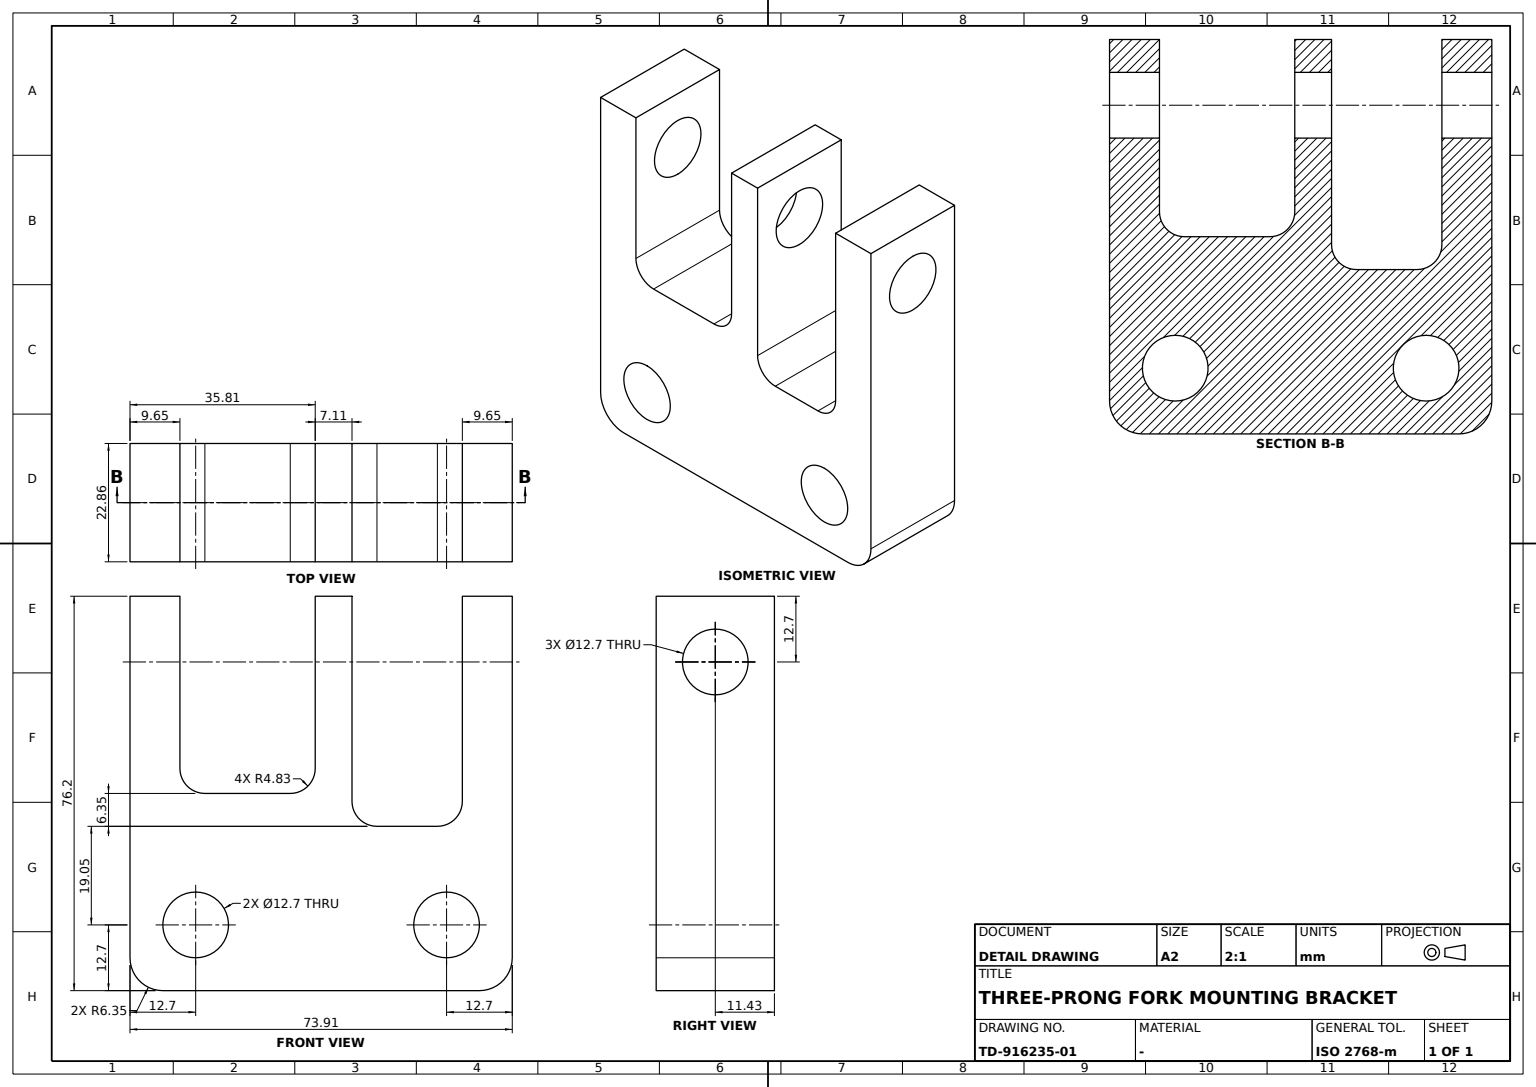
ISO-10303-21;
HEADER;
FILE_DESCRIPTION((''),'2;1');
FILE_NAME('','',(''),(''),'','','');
FILE_SCHEMA(('AUTOMOTIVE_DESIGN'));
ENDSEC;
DATA;
#1=APPLICATION_CONTEXT('');
#2=PRODUCT_CONTEXT('',#1,'mechanical');
#3=PRODUCT('','','',(#2));
#4=PRODUCT_DEFINITION_FORMATION('','',#3);
#5=PRODUCT_DEFINITION_CONTEXT('',#1,'design');
#6=PRODUCT_DEFINITION('','',#4,#5);
#7=PRODUCT_DEFINITION_SHAPE('','',#6);
#8=(LENGTH_UNIT()NAMED_UNIT(*)SI_UNIT(.MILLI.,.METRE.));
#9=(NAMED_UNIT(*)PLANE_ANGLE_UNIT()SI_UNIT($,.RADIAN.));
#10=(NAMED_UNIT(*)SI_UNIT($,.STERADIAN.)SOLID_ANGLE_UNIT());
#11=UNCERTAINTY_MEASURE_WITH_UNIT(LENGTH_MEASURE(0.005),#8,'distance_accuracy_value','');
#12=(GEOMETRIC_REPRESENTATION_CONTEXT(3)GLOBAL_UNCERTAINTY_ASSIGNED_CONTEXT((#11))GLOBAL_UNIT_ASSIGNED_CONTEXT((#8,#9,#10))REPRESENTATION_CONTEXT('',''));
#13=CARTESIAN_POINT('',(-36.957,0.,19.05));
#14=VERTEX_POINT('',#13);
#15=CARTESIAN_POINT('',(-36.957,0.,31.75));
#16=VERTEX_POINT('',#15);
#17=CARTESIAN_POINT('',(-36.957,0.,25.4));
#18=DIRECTION('',(1.,0.,0.));
#19=DIRECTION('',(0.,0.,-1.));
#20=AXIS2_PLACEMENT_3D('',#17,#18,#19);
#21=CIRCLE('',#20,6.35);
#22=EDGE_CURVE('',#14,#16,#21,.T.);
#23=ORIENTED_EDGE('',*,*,#22,.F.);
#24=CARTESIAN_POINT('',(-27.305,0.,19.05));
#25=VERTEX_POINT('',#24);
#26=CARTESIAN_POINT('',(-54963.043,0.,19.05));
#27=VECTOR('',#18,1000.);
#28=LINE('',#26,#27);
#29=EDGE_CURVE('',#25,#14,#28,.F.);
#30=ORIENTED_EDGE('',*,*,#29,.F.);
#31=CARTESIAN_POINT('',(-27.305,0.,31.75));
#32=VERTEX_POINT('',#31);
#33=CARTESIAN_POINT('',(-27.305,0.,25.4));
#34=DIRECTION('',(-1.,0.,0.));
#35=DIRECTION('',(0.,0.,1.));
#36=AXIS2_PLACEMENT_3D('',#33,#34,#35);
#37=CIRCLE('',#36,6.35);
#38=EDGE_CURVE('',#32,#25,#37,.T.);
#39=ORIENTED_EDGE('',*,*,#38,.F.);
#40=CARTESIAN_POINT('',(-54963.043,0.,31.75));
#41=LINE('',#40,#27);
#42=EDGE_CURVE('',#16,#32,#41,.T.);
#43=ORIENTED_EDGE('',*,*,#42,.F.);
#44=EDGE_LOOP('',(#23,#30,#39,#43));
#45=FACE_BOUND('',#44,.T.);
#46=CARTESIAN_POINT('',(-54963.043,0.,25.4));
#47=AXIS2_PLACEMENT_3D('',#46,#18,#19);
#48=CYLINDRICAL_SURFACE('',#47,6.35);
#49=ADVANCED_FACE('',(#45),#48,.F.);
#50=CARTESIAN_POINT('',(-30.607,-11.43,-38.1));
#51=VERTEX_POINT('',#50);
#52=CARTESIAN_POINT('',(-30.607,11.43,-38.1));
#53=VERTEX_POINT('',#52);
#54=DIRECTION('',(0.,1.,0.));
#55=VECTOR('',#54,1000.);
#56=LINE('',#50,#55);
#57=EDGE_CURVE('',#51,#53,#56,.T.);
#58=ORIENTED_EDGE('',*,*,#57,.F.);
#59=CARTESIAN_POINT('',(-36.957,-11.43,-31.75));
#60=VERTEX_POINT('',#59);
#61=CARTESIAN_POINT('',(-30.607,-11.43,-31.75));
#62=DIRECTION('',(0.,-1.,0.));
#63=AXIS2_PLACEMENT_3D('',#61,#62,#19);
#64=CIRCLE('',#63,6.35);
#65=EDGE_CURVE('',#60,#51,#64,.T.);
#66=ORIENTED_EDGE('',*,*,#65,.F.);
#67=CARTESIAN_POINT('',(-36.957,11.43,-31.75));
#68=VERTEX_POINT('',#67);
#69=VECTOR('',#62,1000.);
#70=LINE('',#59,#69);
#71=EDGE_CURVE('',#68,#60,#70,.T.);
#72=ORIENTED_EDGE('',*,*,#71,.F.);
#73=CARTESIAN_POINT('',(-30.607,11.43,-31.75));
#74=AXIS2_PLACEMENT_3D('',#73,#54,#19);
#75=CIRCLE('',#74,6.35);
#76=EDGE_CURVE('',#53,#68,#75,.T.);
#77=ORIENTED_EDGE('',*,*,#76,.F.);
#78=EDGE_LOOP('',(#58,#66,#72,#77));
#79=FACE_BOUND('',#78,.T.);
#80=AXIS2_PLACEMENT_3D('',#61,#54,#35);
#81=CYLINDRICAL_SURFACE('',#80,6.35);
#82=ADVANCED_FACE('',(#79),#81,.T.);
#83=CARTESIAN_POINT('',(30.607,11.43,-38.1));
#84=VERTEX_POINT('',#83);
#85=CARTESIAN_POINT('',(30.607,-11.43,-38.1));
#86=VERTEX_POINT('',#85);
#87=LINE('',#85,#69);
#88=EDGE_CURVE('',#84,#86,#87,.T.);
#89=ORIENTED_EDGE('',*,*,#88,.T.);
#90=CARTESIAN_POINT('',(-36.957,-11.43,-38.1));
#91=LINE('',#90,#27);
#92=EDGE_CURVE('',#51,#86,#91,.T.);
#93=ORIENTED_EDGE('',*,*,#92,.F.);
#94=ORIENTED_EDGE('',*,*,#57,.T.);
#95=CARTESIAN_POINT('',(-36.957,11.43,-38.1));
#96=LINE('',#95,#27);
#97=EDGE_CURVE('',#53,#84,#96,.T.);
#98=ORIENTED_EDGE('',*,*,#97,.T.);
#99=EDGE_LOOP('',(#89,#93,#94,#98));
#100=FACE_BOUND('',#99,.T.);
#101=AXIS2_PLACEMENT_3D('',#90,#35,#18);
#102=PLANE('',#101);
#103=ADVANCED_FACE('',(#100),#102,.F.);
#104=CARTESIAN_POINT('',(-24.257,11.43,-31.75));
#105=VERTEX_POINT('',#104);
#106=CARTESIAN_POINT('',(-24.257,11.43,-19.05));
#107=VERTEX_POINT('',#106);
#108=CARTESIAN_POINT('',(-24.257,11.43,-25.4));
#109=AXIS2_PLACEMENT_3D('',#108,#62,#18);
#110=CIRCLE('',#109,6.35);
#111=EDGE_CURVE('',#105,#107,#110,.T.);
#112=ORIENTED_EDGE('',*,*,#111,.F.);
#113=CARTESIAN_POINT('',(-24.257,-11.43,-31.75));
#114=VERTEX_POINT('',#113);
#115=LINE('',#104,#69);
#116=EDGE_CURVE('',#105,#114,#115,.T.);
#117=ORIENTED_EDGE('',*,*,#116,.T.);
#118=CARTESIAN_POINT('',(-24.257,-11.43,-19.05));
#119=VERTEX_POINT('',#118);
#120=CARTESIAN_POINT('',(-24.257,-11.43,-25.4));
#121=AXIS2_PLACEMENT_3D('',#120,#62,#18);
#122=CIRCLE('',#121,6.35);
#123=EDGE_CURVE('',#114,#119,#122,.T.);
#124=ORIENTED_EDGE('',*,*,#123,.T.);
#125=LINE('',#106,#69);
#126=EDGE_CURVE('',#119,#107,#125,.F.);
#127=ORIENTED_EDGE('',*,*,#126,.T.);
#128=EDGE_LOOP('',(#112,#117,#124,#127));
#129=FACE_BOUND('',#128,.T.);
#130=AXIS2_PLACEMENT_3D('',#108,#62,#19);
#131=CYLINDRICAL_SURFACE('',#130,6.35);
#132=ADVANCED_FACE('',(#129),#131,.F.);
#133=ORIENTED_EDGE('',*,*,#116,.F.);
#134=EDGE_CURVE('',#107,#105,#110,.T.);
#135=ORIENTED_EDGE('',*,*,#134,.F.);
#136=ORIENTED_EDGE('',*,*,#126,.F.);
#137=EDGE_CURVE('',#119,#114,#122,.T.);
#138=ORIENTED_EDGE('',*,*,#137,.T.);
#139=EDGE_LOOP('',(#133,#135,#136,#138));
#140=FACE_BOUND('',#139,.T.);
#141=ADVANCED_FACE('',(#140),#131,.F.);
#142=CARTESIAN_POINT('',(5.969,11.43,38.1));
#143=VERTEX_POINT('',#142);
#144=CARTESIAN_POINT('',(5.969,11.43,-1.524));
#145=VERTEX_POINT('',#144);
#146=VECTOR('',#19,1000.);
#147=LINE('',#142,#146);
#148=EDGE_CURVE('',#143,#145,#147,.T.);
#149=ORIENTED_EDGE('',*,*,#148,.F.);
#150=CARTESIAN_POINT('',(5.969,-11.43,38.1));
#151=VERTEX_POINT('',#150);
#152=LINE('',#142,#69);
#153=EDGE_CURVE('',#143,#151,#152,.T.);
#154=ORIENTED_EDGE('',*,*,#153,.T.);
#155=CARTESIAN_POINT('',(5.969,-11.43,-1.524));
#156=VERTEX_POINT('',#155);
#157=LINE('',#150,#146);
#158=EDGE_CURVE('',#151,#156,#157,.T.);
#159=ORIENTED_EDGE('',*,*,#158,.T.);
#160=LINE('',#144,#55);
#161=EDGE_CURVE('',#156,#145,#160,.T.);
#162=ORIENTED_EDGE('',*,*,#161,.T.);
#163=EDGE_LOOP('',(#149,#154,#159,#162));
#164=FACE_BOUND('',#163,.T.);
#165=CARTESIAN_POINT('',(5.969,0.,31.75));
#166=VERTEX_POINT('',#165);
#167=CARTESIAN_POINT('',(5.969,0.,19.05));
#168=VERTEX_POINT('',#167);
#169=CARTESIAN_POINT('',(5.969,0.,25.4));
#170=AXIS2_PLACEMENT_3D('',#169,#34,#35);
#171=CIRCLE('',#170,6.35);
#172=EDGE_CURVE('',#166,#168,#171,.T.);
#173=ORIENTED_EDGE('',*,*,#172,.T.);
#174=EDGE_CURVE('',#168,#166,#171,.T.);
#175=ORIENTED_EDGE('',*,*,#174,.T.);
#176=EDGE_LOOP('',(#173,#175));
#177=FACE_BOUND('',#176,.T.);
#178=AXIS2_PLACEMENT_3D('',#142,#34,#35);
#179=PLANE('',#178);
#180=ADVANCED_FACE('',(#164,#177),#179,.F.);
#181=ORIENTED_EDGE('',*,*,#88,.F.);
#182=CARTESIAN_POINT('',(36.957,11.43,-31.75));
#183=VERTEX_POINT('',#182);
#184=CARTESIAN_POINT('',(30.607,11.43,-31.75));
#185=AXIS2_PLACEMENT_3D('',#184,#54,#19);
#186=CIRCLE('',#185,6.35);
#187=EDGE_CURVE('',#183,#84,#186,.T.);
#188=ORIENTED_EDGE('',*,*,#187,.F.);
#189=CARTESIAN_POINT('',(36.957,-11.43,-31.75));
#190=VERTEX_POINT('',#189);
#191=LINE('',#189,#55);
#192=EDGE_CURVE('',#190,#183,#191,.T.);
#193=ORIENTED_EDGE('',*,*,#192,.F.);
#194=CARTESIAN_POINT('',(30.607,-11.43,-31.75));
#195=AXIS2_PLACEMENT_3D('',#194,#62,#19);
#196=CIRCLE('',#195,6.35);
#197=EDGE_CURVE('',#86,#190,#196,.T.);
#198=ORIENTED_EDGE('',*,*,#197,.F.);
#199=EDGE_LOOP('',(#181,#188,#193,#198));
#200=FACE_BOUND('',#199,.T.);
#201=AXIS2_PLACEMENT_3D('',#194,#54,#35);
#202=CYLINDRICAL_SURFACE('',#201,6.35);
#203=ADVANCED_FACE('',(#200),#202,.T.);
#204=CARTESIAN_POINT('',(-1.143,11.43,4.826));
#205=VERTEX_POINT('',#204);
#206=CARTESIAN_POINT('',(-1.143,-11.43,4.826));
#207=VERTEX_POINT('',#206);
#208=LINE('',#206,#69);
#209=EDGE_CURVE('',#205,#207,#208,.T.);
#210=ORIENTED_EDGE('',*,*,#209,.F.);
#211=CARTESIAN_POINT('',(-5.969,11.43,0.));
#212=VERTEX_POINT('',#211);
#213=CARTESIAN_POINT('',(-5.969,11.43,4.826));
#214=AXIS2_PLACEMENT_3D('',#213,#62,#19);
#215=CIRCLE('',#214,4.826);
#216=EDGE_CURVE('',#212,#205,#215,.T.);
#217=ORIENTED_EDGE('',*,*,#216,.F.);
#218=CARTESIAN_POINT('',(-5.969,-11.43,0.));
#219=VERTEX_POINT('',#218);
#220=LINE('',#211,#55);
#221=EDGE_CURVE('',#219,#212,#220,.T.);
#222=ORIENTED_EDGE('',*,*,#221,.F.);
#223=CARTESIAN_POINT('',(-5.969,-11.43,4.826));
#224=AXIS2_PLACEMENT_3D('',#223,#54,#19);
#225=CIRCLE('',#224,4.826);
#226=EDGE_CURVE('',#207,#219,#225,.T.);
#227=ORIENTED_EDGE('',*,*,#226,.F.);
#228=EDGE_LOOP('',(#210,#217,#222,#227));
#229=FACE_BOUND('',#228,.T.);
#230=CYLINDRICAL_SURFACE('',#214,4.826);
#231=ADVANCED_FACE('',(#229),#230,.F.);
#232=CARTESIAN_POINT('',(-1.143,0.,19.05));
#233=VERTEX_POINT('',#232);
#234=EDGE_CURVE('',#168,#233,#28,.F.);
#235=ORIENTED_EDGE('',*,*,#234,.F.);
#236=ORIENTED_EDGE('',*,*,#172,.F.);
#237=CARTESIAN_POINT('',(-1.143,0.,31.75));
#238=VERTEX_POINT('',#237);
#239=EDGE_CURVE('',#238,#166,#41,.T.);
#240=ORIENTED_EDGE('',*,*,#239,.F.);
#241=CARTESIAN_POINT('',(-1.143,0.,25.4));
#242=AXIS2_PLACEMENT_3D('',#241,#18,#19);
#243=CIRCLE('',#242,6.35);
#244=EDGE_CURVE('',#233,#238,#243,.T.);
#245=ORIENTED_EDGE('',*,*,#244,.F.);
#246=EDGE_LOOP('',(#235,#236,#240,#245));
#247=FACE_BOUND('',#246,.T.);
#248=ADVANCED_FACE('',(#247),#48,.F.);
#249=CARTESIAN_POINT('',(-22.479,-11.43,0.));
#250=VERTEX_POINT('',#249);
#251=CARTESIAN_POINT('',(-27.305,-11.43,0.));
#252=LINE('',#251,#27);
#253=EDGE_CURVE('',#250,#219,#252,.T.);
#254=ORIENTED_EDGE('',*,*,#253,.T.);
#255=ORIENTED_EDGE('',*,*,#221,.T.);
#256=CARTESIAN_POINT('',(-22.479,11.43,0.));
#257=VERTEX_POINT('',#256);
#258=CARTESIAN_POINT('',(-27.305,11.43,0.));
#259=LINE('',#258,#27);
#260=EDGE_CURVE('',#257,#212,#259,.T.);
#261=ORIENTED_EDGE('',*,*,#260,.F.);
#262=LINE('',#249,#69);
#263=EDGE_CURVE('',#257,#250,#262,.T.);
#264=ORIENTED_EDGE('',*,*,#263,.T.);
#265=EDGE_LOOP('',(#254,#255,#261,#264));
#266=FACE_BOUND('',#265,.T.);
#267=AXIS2_PLACEMENT_3D('',#258,#19,#34);
#268=PLANE('',#267);
#269=ADVANCED_FACE('',(#266),#268,.F.);
#270=CARTESIAN_POINT('',(27.305,11.43,-1.524));
#271=VERTEX_POINT('',#270);
#272=CARTESIAN_POINT('',(27.305,-11.43,-1.524));
#273=VERTEX_POINT('',#272);
#274=LINE('',#272,#69);
#275=EDGE_CURVE('',#271,#273,#274,.T.);
#276=ORIENTED_EDGE('',*,*,#275,.F.);
#277=CARTESIAN_POINT('',(22.479,11.43,-6.35));
#278=VERTEX_POINT('',#277);
#279=CARTESIAN_POINT('',(22.479,11.43,-1.524));
#280=AXIS2_PLACEMENT_3D('',#279,#62,#19);
#281=CIRCLE('',#280,4.826);
#282=EDGE_CURVE('',#278,#271,#281,.T.);
#283=ORIENTED_EDGE('',*,*,#282,.F.);
#284=CARTESIAN_POINT('',(22.479,-11.43,-6.35));
#285=VERTEX_POINT('',#284);
#286=LINE('',#277,#55);
#287=EDGE_CURVE('',#285,#278,#286,.T.);
#288=ORIENTED_EDGE('',*,*,#287,.F.);
#289=CARTESIAN_POINT('',(22.479,-11.43,-1.524));
#290=AXIS2_PLACEMENT_3D('',#289,#54,#19);
#291=CIRCLE('',#290,4.826);
#292=EDGE_CURVE('',#273,#285,#291,.T.);
#293=ORIENTED_EDGE('',*,*,#292,.F.);
#294=EDGE_LOOP('',(#276,#283,#288,#293));
#295=FACE_BOUND('',#294,.T.);
#296=CYLINDRICAL_SURFACE('',#280,4.826);
#297=ADVANCED_FACE('',(#295),#296,.F.);
#298=CARTESIAN_POINT('',(27.305,0.,19.05));
#299=VERTEX_POINT('',#298);
#300=CARTESIAN_POINT('',(36.957,0.,19.05));
#301=VERTEX_POINT('',#300);
#302=EDGE_CURVE('',#299,#301,#28,.T.);
#303=ORIENTED_EDGE('',*,*,#302,.F.);
#304=CARTESIAN_POINT('',(27.305,0.,31.75));
#305=VERTEX_POINT('',#304);
#306=CARTESIAN_POINT('',(27.305,0.,25.4));
#307=AXIS2_PLACEMENT_3D('',#306,#18,#19);
#308=CIRCLE('',#307,6.35);
#309=EDGE_CURVE('',#305,#299,#308,.T.);
#310=ORIENTED_EDGE('',*,*,#309,.F.);
#311=CARTESIAN_POINT('',(36.957,0.,31.75));
#312=VERTEX_POINT('',#311);
#313=EDGE_CURVE('',#312,#305,#41,.F.);
#314=ORIENTED_EDGE('',*,*,#313,.F.);
#315=CARTESIAN_POINT('',(36.957,0.,25.4));
#316=AXIS2_PLACEMENT_3D('',#315,#18,#54);
#317=CIRCLE('',#316,6.35);
#318=EDGE_CURVE('',#312,#301,#317,.T.);
#319=ORIENTED_EDGE('',*,*,#318,.T.);
#320=EDGE_LOOP('',(#303,#310,#314,#319));
#321=FACE_BOUND('',#320,.T.);
#322=ADVANCED_FACE('',(#321),#48,.F.);
#323=CARTESIAN_POINT('',(-36.957,11.43,38.1));
#324=VERTEX_POINT('',#323);
#325=LINE('',#323,#146);
#326=EDGE_CURVE('',#324,#68,#325,.T.);
#327=ORIENTED_EDGE('',*,*,#326,.T.);
#328=ORIENTED_EDGE('',*,*,#71,.T.);
#329=CARTESIAN_POINT('',(-36.957,-11.43,38.1));
#330=VERTEX_POINT('',#329);
#331=LINE('',#329,#146);
#332=EDGE_CURVE('',#330,#60,#331,.T.);
#333=ORIENTED_EDGE('',*,*,#332,.F.);
#334=LINE('',#329,#55);
#335=EDGE_CURVE('',#330,#324,#334,.T.);
#336=ORIENTED_EDGE('',*,*,#335,.T.);
#337=EDGE_LOOP('',(#327,#328,#333,#336));
#338=FACE_BOUND('',#337,.T.);
#339=ORIENTED_EDGE('',*,*,#22,.T.);
#340=EDGE_CURVE('',#16,#14,#21,.T.);
#341=ORIENTED_EDGE('',*,*,#340,.T.);
#342=EDGE_LOOP('',(#339,#341));
#343=FACE_BOUND('',#342,.T.);
#344=AXIS2_PLACEMENT_3D('',#329,#18,#19);
#345=PLANE('',#344);
#346=ADVANCED_FACE('',(#338,#343),#345,.F.);
#347=CARTESIAN_POINT('',(24.257,11.43,-19.05));
#348=VERTEX_POINT('',#347);
#349=CARTESIAN_POINT('',(24.257,-11.43,-19.05));
#350=VERTEX_POINT('',#349);
#351=LINE('',#347,#69);
#352=EDGE_CURVE('',#348,#350,#351,.T.);
#353=ORIENTED_EDGE('',*,*,#352,.T.);
#354=CARTESIAN_POINT('',(24.257,-11.43,-31.75));
#355=VERTEX_POINT('',#354);
#356=CARTESIAN_POINT('',(24.257,-11.43,-25.4));
#357=AXIS2_PLACEMENT_3D('',#356,#62,#18);
#358=CIRCLE('',#357,6.35);
#359=EDGE_CURVE('',#350,#355,#358,.T.);
#360=ORIENTED_EDGE('',*,*,#359,.T.);
#361=CARTESIAN_POINT('',(24.257,11.43,-31.75));
#362=VERTEX_POINT('',#361);
#363=LINE('',#361,#69);
#364=EDGE_CURVE('',#355,#362,#363,.F.);
#365=ORIENTED_EDGE('',*,*,#364,.T.);
#366=CARTESIAN_POINT('',(24.257,11.43,-25.4));
#367=AXIS2_PLACEMENT_3D('',#366,#62,#18);
#368=CIRCLE('',#367,6.35);
#369=EDGE_CURVE('',#348,#362,#368,.T.);
#370=ORIENTED_EDGE('',*,*,#369,.F.);
#371=EDGE_LOOP('',(#353,#360,#365,#370));
#372=FACE_BOUND('',#371,.T.);
#373=AXIS2_PLACEMENT_3D('',#366,#62,#19);
#374=CYLINDRICAL_SURFACE('',#373,6.35);
#375=ADVANCED_FACE('',(#372),#374,.F.);
#376=ORIENTED_EDGE('',*,*,#313,.T.);
#377=EDGE_CURVE('',#299,#305,#308,.T.);
#378=ORIENTED_EDGE('',*,*,#377,.F.);
#379=ORIENTED_EDGE('',*,*,#302,.T.);
#380=EDGE_CURVE('',#301,#312,#317,.T.);
#381=ORIENTED_EDGE('',*,*,#380,.T.);
#382=EDGE_LOOP('',(#376,#378,#379,#381));
#383=FACE_BOUND('',#382,.T.);
#384=ADVANCED_FACE('',(#383),#48,.F.);
#385=ORIENTED_EDGE('',*,*,#209,.T.);
#386=CARTESIAN_POINT('',(-1.143,-11.43,38.1));
#387=VERTEX_POINT('',#386);
#388=CARTESIAN_POINT('',(-1.143,-11.43,0.));
#389=VECTOR('',#35,1000.);
#390=LINE('',#388,#389);
#391=EDGE_CURVE('',#207,#387,#390,.T.);
#392=ORIENTED_EDGE('',*,*,#391,.T.);
#393=CARTESIAN_POINT('',(-1.143,11.43,38.1));
#394=VERTEX_POINT('',#393);
#395=LINE('',#393,#69);
#396=EDGE_CURVE('',#394,#387,#395,.T.);
#397=ORIENTED_EDGE('',*,*,#396,.F.);
#398=CARTESIAN_POINT('',(-1.143,11.43,0.));
#399=LINE('',#398,#389);
#400=EDGE_CURVE('',#205,#394,#399,.T.);
#401=ORIENTED_EDGE('',*,*,#400,.F.);
#402=EDGE_LOOP('',(#385,#392,#397,#401));
#403=FACE_BOUND('',#402,.T.);
#404=EDGE_CURVE('',#238,#233,#243,.T.);
#405=ORIENTED_EDGE('',*,*,#404,.T.);
#406=ORIENTED_EDGE('',*,*,#244,.T.);
#407=EDGE_LOOP('',(#405,#406));
#408=FACE_BOUND('',#407,.T.);
#409=AXIS2_PLACEMENT_3D('',#398,#18,#19);
#410=PLANE('',#409);
#411=ADVANCED_FACE('',(#403,#408),#410,.F.);
#412=ORIENTED_EDGE('',*,*,#161,.F.);
#413=CARTESIAN_POINT('',(10.795,-11.43,-6.35));
#414=VERTEX_POINT('',#413);
#415=CARTESIAN_POINT('',(10.795,-11.43,-1.524));
#416=AXIS2_PLACEMENT_3D('',#415,#54,#19);
#417=CIRCLE('',#416,4.826);
#418=EDGE_CURVE('',#414,#156,#417,.T.);
#419=ORIENTED_EDGE('',*,*,#418,.F.);
#420=CARTESIAN_POINT('',(10.795,11.43,-6.35));
#421=VERTEX_POINT('',#420);
#422=LINE('',#413,#69);
#423=EDGE_CURVE('',#421,#414,#422,.T.);
#424=ORIENTED_EDGE('',*,*,#423,.F.);
#425=CARTESIAN_POINT('',(10.795,11.43,-1.524));
#426=AXIS2_PLACEMENT_3D('',#425,#62,#19);
#427=CIRCLE('',#426,4.826);
#428=EDGE_CURVE('',#145,#421,#427,.T.);
#429=ORIENTED_EDGE('',*,*,#428,.F.);
#430=EDGE_LOOP('',(#412,#419,#424,#429));
#431=FACE_BOUND('',#430,.T.);
#432=CYLINDRICAL_SURFACE('',#426,4.826);
#433=ADVANCED_FACE('',(#431),#432,.F.);
#434=CARTESIAN_POINT('',(-27.305,11.43,4.826));
#435=VERTEX_POINT('',#434);
#436=CARTESIAN_POINT('',(-22.479,11.43,4.826));
#437=AXIS2_PLACEMENT_3D('',#436,#62,#19);
#438=CIRCLE('',#437,4.826);
#439=EDGE_CURVE('',#435,#257,#438,.T.);
#440=ORIENTED_EDGE('',*,*,#439,.F.);
#441=CARTESIAN_POINT('',(-27.305,-11.43,4.826));
#442=VERTEX_POINT('',#441);
#443=LINE('',#434,#55);
#444=EDGE_CURVE('',#442,#435,#443,.T.);
#445=ORIENTED_EDGE('',*,*,#444,.F.);
#446=CARTESIAN_POINT('',(-22.479,-11.43,4.826));
#447=AXIS2_PLACEMENT_3D('',#446,#54,#19);
#448=CIRCLE('',#447,4.826);
#449=EDGE_CURVE('',#250,#442,#448,.T.);
#450=ORIENTED_EDGE('',*,*,#449,.F.);
#451=ORIENTED_EDGE('',*,*,#263,.F.);
#452=EDGE_LOOP('',(#440,#445,#450,#451));
#453=FACE_BOUND('',#452,.T.);
#454=CYLINDRICAL_SURFACE('',#437,4.826);
#455=ADVANCED_FACE('',(#453),#454,.F.);
#456=ORIENTED_EDGE('',*,*,#29,.T.);
#457=ORIENTED_EDGE('',*,*,#340,.F.);
#458=ORIENTED_EDGE('',*,*,#42,.T.);
#459=EDGE_CURVE('',#25,#32,#37,.T.);
#460=ORIENTED_EDGE('',*,*,#459,.F.);
#461=EDGE_LOOP('',(#456,#457,#458,#460));
#462=FACE_BOUND('',#461,.T.);
#463=ADVANCED_FACE('',(#462),#48,.F.);
#464=CARTESIAN_POINT('',(-27.305,11.43,38.1));
#465=VERTEX_POINT('',#464);
#466=CARTESIAN_POINT('',(36.957,11.43,38.1));
#467=VECTOR('',#34,1000.);
#468=LINE('',#466,#467);
#469=EDGE_CURVE('',#465,#324,#468,.T.);
#470=ORIENTED_EDGE('',*,*,#469,.T.);
#471=ORIENTED_EDGE('',*,*,#335,.F.);
#472=CARTESIAN_POINT('',(-27.305,-11.43,38.1));
#473=VERTEX_POINT('',#472);
#474=CARTESIAN_POINT('',(36.957,-11.43,38.1));
#475=LINE('',#474,#467);
#476=EDGE_CURVE('',#473,#330,#475,.T.);
#477=ORIENTED_EDGE('',*,*,#476,.F.);
#478=LINE('',#464,#69);
#479=EDGE_CURVE('',#465,#473,#478,.T.);
#480=ORIENTED_EDGE('',*,*,#479,.F.);
#481=EDGE_LOOP('',(#470,#471,#477,#480));
#482=FACE_BOUND('',#481,.T.);
#483=AXIS2_PLACEMENT_3D('',#474,#19,#34);
#484=PLANE('',#483);
#485=ADVANCED_FACE('',(#482),#484,.F.);
#486=ORIENTED_EDGE('',*,*,#352,.F.);
#487=EDGE_CURVE('',#362,#348,#368,.T.);
#488=ORIENTED_EDGE('',*,*,#487,.F.);
#489=ORIENTED_EDGE('',*,*,#364,.F.);
#490=EDGE_CURVE('',#355,#350,#358,.T.);
#491=ORIENTED_EDGE('',*,*,#490,.T.);
#492=EDGE_LOOP('',(#486,#488,#489,#491));
#493=FACE_BOUND('',#492,.T.);
#494=ADVANCED_FACE('',(#493),#374,.F.);
#495=VERTEX_POINT('',#474);
#496=VERTEX_POINT('',#466);
#497=LINE('',#474,#55);
#498=EDGE_CURVE('',#495,#496,#497,.T.);
#499=ORIENTED_EDGE('',*,*,#498,.T.);
#500=CARTESIAN_POINT('',(27.305,11.43,38.1));
#501=VERTEX_POINT('',#500);
#502=EDGE_CURVE('',#496,#501,#468,.T.);
#503=ORIENTED_EDGE('',*,*,#502,.T.);
#504=CARTESIAN_POINT('',(27.305,-11.43,38.1));
#505=VERTEX_POINT('',#504);
#506=LINE('',#500,#69);
#507=EDGE_CURVE('',#501,#505,#506,.T.);
#508=ORIENTED_EDGE('',*,*,#507,.T.);
#509=EDGE_CURVE('',#495,#505,#475,.T.);
#510=ORIENTED_EDGE('',*,*,#509,.F.);
#511=EDGE_LOOP('',(#499,#503,#508,#510));
#512=FACE_BOUND('',#511,.T.);
#513=ADVANCED_FACE('',(#512),#484,.F.);
#514=ORIENTED_EDGE('',*,*,#234,.T.);
#515=ORIENTED_EDGE('',*,*,#404,.F.);
#516=ORIENTED_EDGE('',*,*,#239,.T.);
#517=ORIENTED_EDGE('',*,*,#174,.F.);
#518=EDGE_LOOP('',(#514,#515,#516,#517));
#519=FACE_BOUND('',#518,.T.);
#520=ADVANCED_FACE('',(#519),#48,.F.);
#521=CARTESIAN_POINT('',(5.969,11.43,-6.35));
#522=LINE('',#521,#27);
#523=EDGE_CURVE('',#421,#278,#522,.T.);
#524=ORIENTED_EDGE('',*,*,#523,.F.);
#525=ORIENTED_EDGE('',*,*,#423,.T.);
#526=CARTESIAN_POINT('',(5.969,-11.43,-6.35));
#527=LINE('',#526,#27);
#528=EDGE_CURVE('',#414,#285,#527,.T.);
#529=ORIENTED_EDGE('',*,*,#528,.T.);
#530=ORIENTED_EDGE('',*,*,#287,.T.);
#531=EDGE_LOOP('',(#524,#525,#529,#530));
#532=FACE_BOUND('',#531,.T.);
#533=AXIS2_PLACEMENT_3D('',#521,#19,#34);
#534=PLANE('',#533);
#535=ADVANCED_FACE('',(#532),#534,.F.);
#536=ORIENTED_EDGE('',*,*,#396,.T.);
#537=EDGE_CURVE('',#151,#387,#475,.T.);
#538=ORIENTED_EDGE('',*,*,#537,.F.);
#539=ORIENTED_EDGE('',*,*,#153,.F.);
#540=EDGE_CURVE('',#143,#394,#468,.T.);
#541=ORIENTED_EDGE('',*,*,#540,.T.);
#542=EDGE_LOOP('',(#536,#538,#539,#541));
#543=FACE_BOUND('',#542,.T.);
#544=ADVANCED_FACE('',(#543),#484,.F.);
#545=CARTESIAN_POINT('',(27.305,11.43,-6.35));
#546=LINE('',#545,#389);
#547=EDGE_CURVE('',#271,#501,#546,.T.);
#548=ORIENTED_EDGE('',*,*,#547,.F.);
#549=ORIENTED_EDGE('',*,*,#275,.T.);
#550=CARTESIAN_POINT('',(27.305,-11.43,-6.35));
#551=LINE('',#550,#389);
#552=EDGE_CURVE('',#273,#505,#551,.T.);
#553=ORIENTED_EDGE('',*,*,#552,.T.);
#554=ORIENTED_EDGE('',*,*,#507,.F.);
#555=EDGE_LOOP('',(#548,#549,#553,#554));
#556=FACE_BOUND('',#555,.T.);
#557=ORIENTED_EDGE('',*,*,#309,.T.);
#558=ORIENTED_EDGE('',*,*,#377,.T.);
#559=EDGE_LOOP('',(#557,#558));
#560=FACE_BOUND('',#559,.T.);
#561=AXIS2_PLACEMENT_3D('',#545,#18,#19);
#562=PLANE('',#561);
#563=ADVANCED_FACE('',(#556,#560),#562,.F.);
#564=ORIENTED_EDGE('',*,*,#111,.T.);
#565=ORIENTED_EDGE('',*,*,#134,.T.);
#566=EDGE_LOOP('',(#564,#565));
#567=FACE_BOUND('',#566,.T.);
#568=ORIENTED_EDGE('',*,*,#439,.T.);
#569=ORIENTED_EDGE('',*,*,#260,.T.);
#570=ORIENTED_EDGE('',*,*,#216,.T.);
#571=ORIENTED_EDGE('',*,*,#400,.T.);
#572=ORIENTED_EDGE('',*,*,#540,.F.);
#573=ORIENTED_EDGE('',*,*,#148,.T.);
#574=ORIENTED_EDGE('',*,*,#428,.T.);
#575=ORIENTED_EDGE('',*,*,#523,.T.);
#576=ORIENTED_EDGE('',*,*,#282,.T.);
#577=ORIENTED_EDGE('',*,*,#547,.T.);
#578=ORIENTED_EDGE('',*,*,#502,.F.);
#579=CARTESIAN_POINT('',(36.957,11.43,-38.1));
#580=LINE('',#579,#389);
#581=EDGE_CURVE('',#183,#496,#580,.T.);
#582=ORIENTED_EDGE('',*,*,#581,.F.);
#583=ORIENTED_EDGE('',*,*,#187,.T.);
#584=ORIENTED_EDGE('',*,*,#97,.F.);
#585=ORIENTED_EDGE('',*,*,#76,.T.);
#586=ORIENTED_EDGE('',*,*,#326,.F.);
#587=ORIENTED_EDGE('',*,*,#469,.F.);
#588=LINE('',#464,#146);
#589=EDGE_CURVE('',#465,#435,#588,.T.);
#590=ORIENTED_EDGE('',*,*,#589,.T.);
#591=EDGE_LOOP('',(#568,#569,#570,#571,#572,#573,#574,#575,#576,#577,#578,#582,#583,#584,#585,#586,#587,#590));
#592=FACE_BOUND('',#591,.T.);
#593=ORIENTED_EDGE('',*,*,#369,.T.);
#594=ORIENTED_EDGE('',*,*,#487,.T.);
#595=EDGE_LOOP('',(#593,#594));
#596=FACE_BOUND('',#595,.T.);
#597=CARTESIAN_POINT('',(0.,11.43,0.));
#598=AXIS2_PLACEMENT_3D('',#597,#62,#19);
#599=PLANE('',#598);
#600=ADVANCED_FACE('',(#567,#592,#596),#599,.F.);
#601=ORIENTED_EDGE('',*,*,#459,.T.);
#602=ORIENTED_EDGE('',*,*,#38,.T.);
#603=EDGE_LOOP('',(#601,#602));
#604=FACE_BOUND('',#603,.T.);
#605=ORIENTED_EDGE('',*,*,#589,.F.);
#606=ORIENTED_EDGE('',*,*,#479,.T.);
#607=LINE('',#472,#146);
#608=EDGE_CURVE('',#473,#442,#607,.T.);
#609=ORIENTED_EDGE('',*,*,#608,.T.);
#610=ORIENTED_EDGE('',*,*,#444,.T.);
#611=EDGE_LOOP('',(#605,#606,#609,#610));
#612=FACE_BOUND('',#611,.T.);
#613=AXIS2_PLACEMENT_3D('',#464,#34,#35);
#614=PLANE('',#613);
#615=ADVANCED_FACE('',(#604,#612),#614,.F.);
#616=ORIENTED_EDGE('',*,*,#509,.T.);
#617=ORIENTED_EDGE('',*,*,#552,.F.);
#618=ORIENTED_EDGE('',*,*,#292,.T.);
#619=ORIENTED_EDGE('',*,*,#528,.F.);
#620=ORIENTED_EDGE('',*,*,#418,.T.);
#621=ORIENTED_EDGE('',*,*,#158,.F.);
#622=ORIENTED_EDGE('',*,*,#537,.T.);
#623=ORIENTED_EDGE('',*,*,#391,.F.);
#624=ORIENTED_EDGE('',*,*,#226,.T.);
#625=ORIENTED_EDGE('',*,*,#253,.F.);
#626=ORIENTED_EDGE('',*,*,#449,.T.);
#627=ORIENTED_EDGE('',*,*,#608,.F.);
#628=ORIENTED_EDGE('',*,*,#476,.T.);
#629=ORIENTED_EDGE('',*,*,#332,.T.);
#630=ORIENTED_EDGE('',*,*,#65,.T.);
#631=ORIENTED_EDGE('',*,*,#92,.T.);
#632=ORIENTED_EDGE('',*,*,#197,.T.);
#633=CARTESIAN_POINT('',(36.957,-11.43,-38.1));
#634=LINE('',#633,#389);
#635=EDGE_CURVE('',#190,#495,#634,.T.);
#636=ORIENTED_EDGE('',*,*,#635,.T.);
#637=EDGE_LOOP('',(#616,#617,#618,#619,#620,#621,#622,#623,#624,#625,#626,#627,#628,#629,#630,#631,#632,#636));
#638=FACE_BOUND('',#637,.T.);
#639=ORIENTED_EDGE('',*,*,#490,.F.);
#640=ORIENTED_EDGE('',*,*,#359,.F.);
#641=EDGE_LOOP('',(#639,#640));
#642=FACE_BOUND('',#641,.T.);
#643=ORIENTED_EDGE('',*,*,#123,.F.);
#644=ORIENTED_EDGE('',*,*,#137,.F.);
#645=EDGE_LOOP('',(#643,#644));
#646=FACE_BOUND('',#645,.T.);
#647=CARTESIAN_POINT('',(0.,-11.43,0.));
#648=AXIS2_PLACEMENT_3D('',#647,#62,#19);
#649=PLANE('',#648);
#650=ADVANCED_FACE('',(#638,#642,#646),#649,.T.);
#651=ORIENTED_EDGE('',*,*,#192,.T.);
#652=ORIENTED_EDGE('',*,*,#581,.T.);
#653=ORIENTED_EDGE('',*,*,#498,.F.);
#654=ORIENTED_EDGE('',*,*,#635,.F.);
#655=EDGE_LOOP('',(#651,#652,#653,#654));
#656=FACE_BOUND('',#655,.T.);
#657=ORIENTED_EDGE('',*,*,#380,.F.);
#658=ORIENTED_EDGE('',*,*,#318,.F.);
#659=EDGE_LOOP('',(#657,#658));
#660=FACE_BOUND('',#659,.T.);
#661=AXIS2_PLACEMENT_3D('',#633,#34,#35);
#662=PLANE('',#661);
#663=ADVANCED_FACE('',(#656,#660),#662,.F.);
#664=CLOSED_SHELL('',(#49,#82,#103,#132,#141,#180,#203,#231,#248,#269,#297,#322,#346,#375,#384,#411,#433,#455,#463,#485,#494,#513,#520,#535,#544,#563,#600,#615,#650,#663));
#665=MANIFOLD_SOLID_BREP('',#664);
#666=ADVANCED_BREP_SHAPE_REPRESENTATION('',(#665),#12);
#667=SHAPE_DEFINITION_REPRESENTATION(#7,#666);
ENDSEC;
END-ISO-10303-21;
